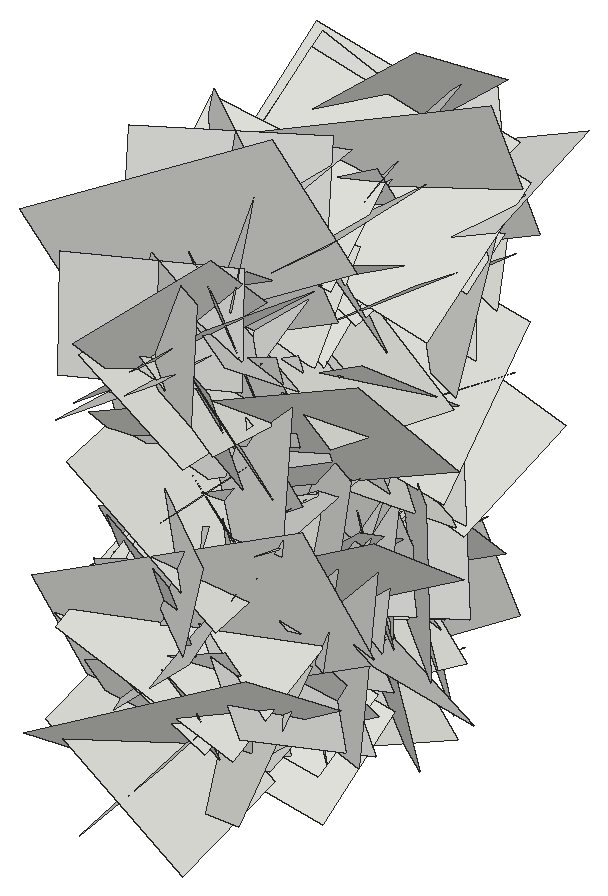
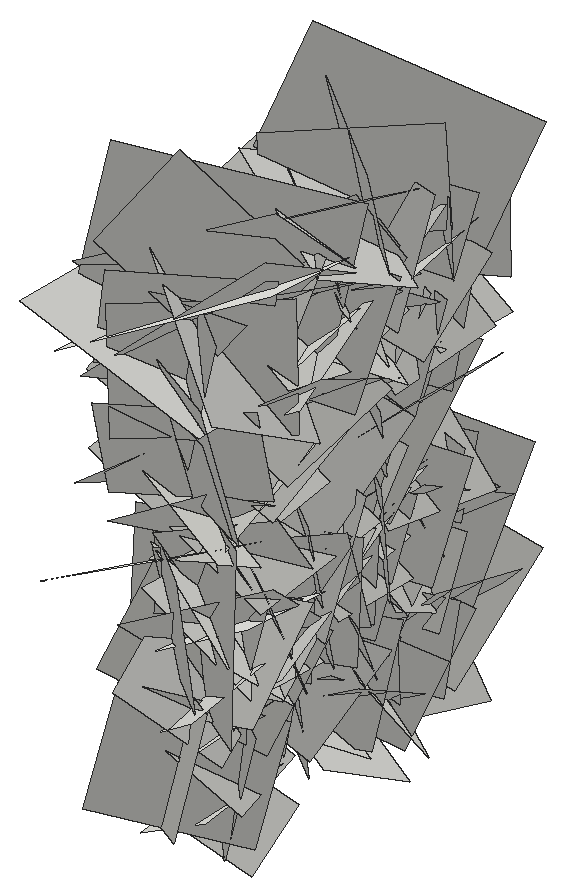
# SketchUp Ruby script. Lengths in inches.
U = 1.inch
M = Sketchup.active_model
def pt(a) = Geom::Point3d.new(a.map { |v| v * U })
def face(e, loops, mat)
  f = e.add_face(loops[0].map { |a| pt(a) })
  loops[1..].each { |l| e.add_face(l.map { |a| pt(a) }).erase! }
  f.material = f.back_material = mat if mat
  f
end
# faces: each face lists its corners as indices into pts; further lists are holes
def faces(e, pts, list, mat = nil) = list.each { |f| face(e, (f[0].is_a?(Array) ? f : [f]).map { |l| l.map { |i| pts[i] } }, mat) }
# xy, xz, yz: faces in a plane at the given z, y or x. An outline is a flat list of corners, or four numbers for a rectangle; further outlines are holes
def ring(l) = l.size == 4 ? [[l[0], l[1]], [l[2], l[1]], [l[2], l[3]], [l[0], l[3]]] : l.each_slice(2).to_a
def flat(e, list, mat, &to3) = list.each { |f| face(e, (f[0].is_a?(Array) ? f : [f]).map { |l| ring(l).map { |u, v| to3.(u, v) } }, mat) }
def xy(e, z, list, mat = nil) = flat(e, list, mat) { |x, y| [x, y, z] }
def xz(e, y, list, mat = nil) = flat(e, list, mat) { |x, z| [x, y, z] }
def yz(e, x, list, mat = nil) = flat(e, list, mat) { |y, z| [x, y, z] }
def lines(e, pts, list) = list.each { |a, b| e.add_line(pt(pts[a]), pt(pts[b])) }
# prism: a flat outline (further loops are holes) pulled along v
def prism(e, loops, v, mat = nil)
  f = face(e, loops, mat); d = Geom::Vector3d.new(v.map { |x| x * U })
  f.pushpull(f.normal.samedirection?(d) ? d.length : -d.length)
end
def box(e, o, s, mat = nil) = prism(e, [[o, [o[0] + s[0], o[1], o[2]], [o[0] + s[0], o[1] + s[1], o[2]], [o[0], o[1] + s[1], o[2]]]], [0, 0, s[2]], mat)
def at(x, y, z, deg = 0) = Geom::Transformation.translation(pt([x, y, z])) * Geom::Transformation.rotation(ORIGIN, Z_AXIS, deg.degrees)
def axes(o, x, y, z) = Geom::Transformation.new([*x, 0, *y, 0, *z, 0, *pt(o).to_a, 1])
def part(name) = M.definitions.add(name)
# library, detail: a bought-in or finely detailed component or shape, given as its bounding box
def library(name, o, s) = part(name).tap { |d| box(d.entities, o, s) }
def detail(e, o, s) = box(e.add_group.entities, o, s)
def put(e, d, t, mat = nil) = e.add_instance(d, t).tap { |i| i.material = mat if mat }
def group(e, t, mat = nil) = e.add_group.tap { |g| g.transformation = t; g.material = mat if mat }.entities
root = M.entities
c1 = part("Component\#6")
p = [[0.01,0,0],[0,3.24,4.54],[4.32,3.24,4.54],[4.33,0,0]]
faces(c1.entities,p,[[0,1,2,3]])
put(root,c1,axes([420.52,153.52,29.46],[-0.08102,0.00764,-0.81457],[-0.10707,-0.81193,0.00187],[0.85682,-0.10074,-0.07679]))
put(root,c1,axes([420.52,158.01,30.39],[0.08038,-0.60995,0.00551],[-0.02253,0.00291,0.6143],[0.64618,0.07598,0.02073]))
put(root,c1,axes([420.52,151.89,27.92],[0.07457,-0.37507,-0.49968],[-0.035,-0.50437,0.37394],[0.66135,0.0156,0.07613]))
put(root,c1,axes([424.49,158.65,23.12],[0.03,-0.65446,0.65644],[-0.11713,0.64968,0.65248],[-0.97555,-0.09812,-0.05816]))
put(root,c1,axes([420.52,150.81,32.67],[-0.03105,-0.70657,0.01303],[0.00041,0.01303,0.70717],[0.74909,-0.02929,0.00015]))
put(root,c1,axes([424.49,155.99,38.05],[-0.0315,0.52335,-0.79271],[0.01447,-0.79278,-0.52391],[-1.00678,-0.02777,0.01727]))
put(root,c1,axes([420.52,155.3,36.05],[-0.02231,-0.46484,-0.62566],[-0.10069,-0.6197,0.4636],[0.82005,-0.08874,0.0399]))
put(root,c1,axes([424.49,160.9375,37.33],[-0.13153,0.12633,-0.90974],[0.10231,-0.91113,-0.13969],[-0.96819,-0.11344,0.10882]))
put(root,c1,axes([424.49,153.79,24.7],[0.00565,-0.43188,0.90191],[0.04751,0.90112,0.43124],[-1.05892,0.03812,0.02416]))
put(root,c1,axes([424.49,152.27,30.34],[-0.04267,0.47891,-0.74389],[-0.05776,-0.74459,-0.47642],[-0.93603,0.02411,0.06331]))
put(root,c1,axes([424.49,150.92,33.45],[0.01124,-0.40239,0.85237],[-0.02564,0.85203,0.40253],[-0.99881,-0.0264,-0.00074]))
put(root,c1,axes([420.52,153.82,25.23],[0.04726,-0.11023,0.59197],[0.093,0.58845,0.10297],[0.63147,-0.07841,-0.05947]))
put(root,c1,axes([420.52,149.71,29.1],[0.04042,0.22115,-0.567],[0.10046,-0.56334,-0.21335],[0.63725,0.07479,0.0696]))
put(root,c1,axes([424.49,154.45,36.57],[-0.07713,0.81709,0.22722],[-0.03645,0.22503,-0.82021],[-0.89825,-0.07929,0.01378]))
put(root,c1,axes([420.52,158.75,26.14],[0.12859,0.59437,-0.23179],[-0.06253,-0.22448,-0.60651],[0.67335,-0.13435,-0.01206]))
put(root,c1,axes([424.49,156.72,22.08],[0.00521,-0.94479,0.50901],[0.17637,0.50353,0.93301],[-1.12382,0.07464,0.14878]))
put(root,c1,axes([420.52,156.34,37.48],[-0.20366,-0.78098,-0.33642],[0.07649,-0.35863,0.79133],[0.89812,-0.14656,-0.14368]))
put(root,c1,axes([424.49,150.56,37.37],[-0.01495,0.72639,-0.4873],[-0.06872,-0.48689,-0.7239],[-0.92463,0.02444,0.06168]))
put(root,c1,axes([420.52,156.49,28.09],[0.01227,0.36562,0.53928],[0.0952,0.53332,-0.36351],[0.68404,-0.08079,0.04092]))
put(root,c1,axes([424.49,150.4,30.92],[-0.04252,-0.27759,0.76161],[-0.13298,0.75548,0.26875],[-0.84891,-0.10444,-0.08025]))
put(root,c1,axes([424.49,152.31,24.83],[-0.14132,0.38772,0.61473],[-0.11706,0.60692,-0.40674],[-0.76145,-0.16526,-0.05156]))
put(root,c1,axes([420.52,150.69,21.46],[-0.08617,-0.06424,0.73191],[0.1147,0.7273,0.07585],[0.77031,-0.11548,0.07058]))
put(root,c1,axes([420.52,149.63,26.39],[-0.05575,0.3601,-0.58557],[0.15834,-0.56726,-0.36226],[0.71127,0.15451,0.03475]))
put(root,c1,axes([420.52,153.92,21.15],[-0.0271,-0.2919,0.8704],[-0.20523,0.85287,0.28034],[0.95124,0.17569,0.08528]))
put(root,c1,axes([420.52,159.1875,20.3125],[-0.01409,-0.35632,0.80543],[-0.16766,0.79339,0.34838],[0.91839,0.13938,0.07596]))
put(root,c1,axes([424.49,157.73,31.39],[0.13129,-0.92283,0.37392],[-0.04334,0.37177,0.93107],[-1.05456,-0.13017,0.00829]))
put(root,c1,axes([420.52,147.16,24.1],[-0.03025,0.92414,0.23442],[-0.23339,0.2218,-0.90118],[0.98329,0.08108,-0.20669]))
put(root,c1,axes([420.52,159.76,21.63],[0.09665,-0.666,0.12875],[-0.03078,0.12595,0.67212],[0.71837,0.095,0.01147]))
put(root,c1,axes([424.49,154.61,36.92],[0.07328,1.03426,0.55463],[0.26621,0.52968,-1.01904],[-1.21518,0.17841,-0.1898]))
put(root,c1,axes([420.52,160.84,30.26],[0.09118,-0.56201,-0.30691],[0.0596,-0.30185,0.56849],[0.67615,0.1024,-0.00872]))
put(root,c1,axes([420.52,156.05,22.34],[0.04217,-0.56806,-0.37659],[0.07293,-0.37196,0.56834],[0.71876,0.07107,-0.03557]))
put(root,c1,axes([424.49,158.82,28.52],[0.0834,-0.34729,-0.88838],[-0.00654,-0.89156,0.34799],[-1.01106,-0.02288,-0.07553]))
put(root,c1,axes([424.49,151.53,22],[0.08087,0.78957,0.40941],[-0.10212,0.41583,-0.78401],[-0.93722,0.02282,0.12075]))
put(root,c1,axes([424.49,152.86,25.21],[-0.07237,-0.84668,-0.40971],[0.16913,-0.41526,0.83156],[-0.98259,-0.00911,0.17331]))
put(root,c1,axes([424.49,150.44,37.52],[0.01758,-0.03984,-0.83316],[-0.08726,-0.82933,0.03802],[-0.87984,0.08145,-0.02042]))
put(root,c1,axes([424.49,161.57,34.4],[0.05292,-0.24359,-0.78611],[-0.1523,-0.77804,0.23197],[-0.85897,0.12294,-0.08956]))
put(root,c1,axes([420.52,154.14,39.875],[-0.07687,-0.17009,-0.90128],[-0.07958,-0.89996,0.17589],[0.96896,-0.0874,-0.05706]))
put(root,c1,axes([420.52,159.35,19.53],[0.12506,-0.65018,0.20227],[-0.00025,0.20525,0.65988],[0.72178,0.11273,-0.03482]))
put(root,c1,axes([424.49,155.63,34.51],[0.04715,-0.7148,-0.47013],[-0.06325,-0.47221,0.71232],[-0.90467,-0.00424,-0.0743]))
put(root,c1,axes([424.49,151.43,29.49],[0.01376,0.93036,0.01045],[0.09599,0.00914,-0.92605],[-0.98156,0.01394,-0.09041]))
put(root,c1,axes([424.49,156.02,27.27],[-0.01737,0.78195,0.05447],[-0.0729,0.05284,-0.77921],[-0.82768,-0.02106,0.06749]))
put(root,c1,axes([420.52,152.23,36.27],[0.17612,0.33723,0.58016],[-0.03508,0.60107,-0.33991],[0.71045,-0.05392,-0.16061]))
put(root,c1,axes([420.52,152.86,32.22],[-0.07765,-0.95123,0.12327],[-0.10469,0.13045,0.94796],[1.01133,-0.05954,0.1076]))
put(root,c1,axes([424.49,160.42,26.72],[0.04031,-0.6417,-0.5437],[-0.04231,-0.54502,0.64047],[-0.89052,-0.00315,-0.05504]))
put(root,c1,axes([420.52,153.18,27.99],[-0.08911,-1.01671,-0.11332],[-0.1646,-0.0997,1.00972],[1.07181,-0.09984,0.14565]))
put(root,c1,axes([424.49,153.18,27.99],[0.08911,-1.01671,-0.11332],[0.1646,-0.0997,1.00972],[-1.07181,-0.09984,0.14565]))
put(root,c1,axes([420.52,160.42,26.72],[-0.04031,-0.6417,-0.5437],[0.04231,-0.54502,0.64047],[0.89052,-0.00315,-0.05504]))
put(root,c1,axes([424.49,152.86,32.22],[0.07765,-0.95123,0.12327],[0.10469,0.13045,0.94796],[-1.01133,-0.05954,0.1076]))
put(root,c1,axes([424.49,152.23,36.27],[-0.17612,0.33723,0.58016],[0.03508,0.60107,-0.33991],[-0.71045,-0.05392,-0.16061]))
put(root,c1,axes([420.52,156.02,27.27],[0.01737,0.78195,0.05447],[0.0729,0.05284,-0.77921],[0.82768,-0.02106,0.06749]))
put(root,c1,axes([420.52,151.43,29.49],[-0.01376,0.93036,0.01045],[-0.09599,0.00914,-0.92605],[0.98156,0.01394,-0.09041]))
put(root,c1,axes([420.52,155.63,34.51],[-0.04715,-0.7148,-0.47013],[0.06325,-0.47221,0.71232],[0.90467,-0.00424,-0.0743]))
put(root,c1,axes([424.49,159.35,19.53],[-0.12506,-0.65018,0.20227],[0.00025,0.20525,0.65988],[-0.72178,0.11273,-0.03482]))
put(root,c1,axes([424.49,154.14,39.875],[0.07687,-0.17009,-0.90128],[0.07958,-0.89996,0.17589],[-0.96896,-0.0874,-0.05706]))
put(root,c1,axes([420.52,161.57,34.4],[-0.05292,-0.24359,-0.78611],[0.1523,-0.77804,0.23197],[0.85897,0.12294,-0.08956]))
put(root,c1,axes([420.52,150.44,37.52],[-0.01758,-0.03984,-0.83316],[0.08726,-0.82933,0.03802],[0.87984,0.08145,-0.02042]))
put(root,c1,axes([420.52,152.86,25.21],[0.07237,-0.84668,-0.40971],[-0.16913,-0.41526,0.83156],[0.98259,-0.00911,0.17331]))
put(root,c1,axes([420.52,151.53,22],[-0.08087,0.78957,0.40941],[0.10212,0.41583,-0.78401],[0.93722,0.02282,0.12075]))
put(root,c1,axes([420.52,158.82,28.52],[-0.0834,-0.34729,-0.88838],[0.00654,-0.89156,0.34799],[1.01106,-0.02288,-0.07553]))
put(root,c1,axes([424.49,156.05,22.34],[-0.04217,-0.56806,-0.37659],[-0.07293,-0.37196,0.56834],[-0.71876,0.07107,-0.03557]))
put(root,c1,axes([424.49,160.84,30.26],[-0.09118,-0.56201,-0.30691],[-0.0596,-0.30185,0.56849],[-0.67615,0.1024,-0.00872]))
put(root,c1,axes([420.52,154.61,36.92],[-0.07328,1.03426,0.55463],[-0.26621,0.52968,-1.01904],[1.21518,0.17841,-0.1898]))
put(root,c1,axes([424.49,159.76,21.63],[-0.09665,-0.666,0.12875],[0.03078,0.12595,0.67212],[-0.71837,0.095,0.01147]))
put(root,c1,axes([424.49,147.16,24.1],[0.03025,0.92414,0.23442],[0.23339,0.2218,-0.90118],[-0.98329,0.08108,-0.20669]))
put(root,c1,axes([420.52,157.73,31.39],[-0.13129,-0.92283,0.37392],[0.04334,0.37177,0.93107],[1.05456,-0.13017,0.00829]))
put(root,c1,axes([424.49,159.1875,20.3125],[0.01409,-0.35632,0.80543],[0.16766,0.79339,0.34838],[-0.91839,0.13938,0.07596]))
put(root,c1,axes([424.49,153.92,21.15],[0.0271,-0.2919,0.8704],[0.20523,0.85287,0.28034],[-0.95124,0.17569,0.08528]))
put(root,c1,axes([424.49,149.63,26.39],[0.05575,0.3601,-0.58557],[-0.15834,-0.56726,-0.36226],[-0.71127,0.15451,0.03475]))
put(root,c1,axes([424.49,150.69,21.46],[0.08617,-0.06424,0.73191],[-0.1147,0.7273,0.07585],[-0.77031,-0.11548,0.07058]))
put(root,c1,axes([420.52,152.31,24.83],[0.14132,0.38772,0.61473],[0.11706,0.60692,-0.40674],[0.76145,-0.16526,-0.05156]))
put(root,c1,axes([420.52,150.4,30.92],[0.04252,-0.27759,0.76161],[0.13298,0.75548,0.26875],[0.84891,-0.10444,-0.08025]))
put(root,c1,axes([424.49,156.49,28.09],[-0.01227,0.36562,0.53928],[-0.0952,0.53332,-0.36351],[-0.68404,-0.08079,0.04092]))
put(root,c1,axes([420.52,150.56,37.37],[0.01495,0.72639,-0.4873],[0.06872,-0.48689,-0.7239],[0.92463,0.02444,0.06168]))
put(root,c1,axes([424.49,156.34,37.48],[0.20366,-0.78098,-0.33642],[-0.07649,-0.35863,0.79133],[-0.89812,-0.14656,-0.14368]))
put(root,c1,axes([420.52,156.72,22.08],[-0.00521,-0.94479,0.50901],[-0.17637,0.50353,0.93301],[1.12382,0.07464,0.14878]))
put(root,c1,axes([424.49,158.75,26.14],[-0.12859,0.59437,-0.23179],[0.06253,-0.22448,-0.60651],[-0.67335,-0.13435,-0.01206]))
put(root,c1,axes([420.52,154.45,36.57],[0.07713,0.81709,0.22722],[0.03645,0.22503,-0.82021],[0.89825,-0.07929,0.01378]))
put(root,c1,axes([424.49,149.71,29.1],[-0.04042,0.22115,-0.567],[-0.10046,-0.56334,-0.21335],[-0.63725,0.07479,0.0696]))
put(root,c1,axes([424.49,153.82,25.23],[-0.04726,-0.11023,0.59197],[-0.093,0.58845,0.10297],[-0.63147,-0.07841,-0.05947]))
put(root,c1,axes([420.52,150.92,33.45],[-0.01124,-0.40239,0.85237],[0.02564,0.85203,0.40253],[0.99881,-0.0264,-0.00074]))
put(root,c1,axes([420.52,152.27,30.34],[0.04267,0.47891,-0.74389],[0.05776,-0.74459,-0.47642],[0.93603,0.02411,0.06331]))
put(root,c1,axes([420.52,153.79,24.7],[-0.00565,-0.43188,0.90191],[-0.04751,0.90112,0.43124],[1.05892,0.03812,0.02416]))
put(root,c1,axes([420.52,160.9375,37.33],[0.13153,0.12633,-0.90974],[-0.10231,-0.91113,-0.13969],[0.96819,-0.11344,0.10882]))
put(root,c1,axes([424.49,155.3,36.05],[0.02231,-0.46484,-0.62566],[0.10069,-0.6197,0.4636],[-0.82005,-0.08874,0.0399]))
put(root,c1,axes([420.52,155.99,38.05],[0.0315,0.52335,-0.79271],[-0.01447,-0.79278,-0.52391],[1.00678,-0.02777,0.01727]))
put(root,c1,axes([424.49,150.81,32.67],[0.03105,-0.70657,0.01303],[-0.00041,0.01303,0.70717],[-0.74909,-0.02929,0.00015]))
put(root,c1,axes([420.52,158.65,23.12],[-0.03,-0.65446,0.65644],[0.11713,0.64968,0.65248],[0.97555,-0.09812,-0.05816]))
put(root,c1,axes([424.49,151.89,27.92],[-0.07457,-0.37507,-0.49968],[0.035,-0.50437,0.37394],[-0.66135,0.0156,0.07613]))
put(root,c1,axes([424.49,158.01,30.39],[-0.08038,-0.60995,0.00551],[0.02253,0.00291,0.6143],[-0.64618,0.07598,0.02073]))
put(root,c1,axes([424.49,153.52,29.46],[0.08102,0.00764,-0.81457],[0.10707,-0.81193,0.00187],[-0.85682,-0.10074,-0.07679]))
put(root,c1,axes([420.52,152.65,32.7],[-0.31384,1.21799,0.62272],[-0.13011,0.61092,-1.25326],[1.44417,0.31973,0.02242]))
put(root,c1,axes([420.52,149.65,34.23],[-0.2234,-0.54463,1.08834],[-0.02633,1.10624,0.54877],[1.28976,-0.07175,0.19972]))
put(root,c1,axes([424.49,152.7,33.94],[0.15183,0.13661,-0.74127],[-0.04087,-0.75222,-0.14607],[-0.79793,0.06452,-0.13357]))
put(root,c1,axes([424.49,158.73,27.09],[0.13155,-0.14233,-0.74779],[0.00006,-0.75766,0.14422],[-0.80689,-0.02326,-0.12191]))
put(root,c1,axes([420.52,158.66,27.8],[0.19419,0.10037,-0.91545],[-0.10975,-0.92523,-0.12216],[0.97001,-0.12478,0.16945]))
put(root,c1,axes([424.49,156.65,23.33],[-0.01341,0.01203,0.69899],[0.10657,0.69187,-0.01009],[-0.73333,0.10033,-0.01425]))
put(root,c1,axes([420.52,154.96,37.56],[-0.27688,1.1515,0.31839],[0.11464,0.34737,-1.16756],[1.26119,0.22122,0.17603]))
put(root,c1,axes([420.52,152.42,20.54],[-0.05004,-0.6691,0.77955],[0.05919,0.77755,0.67076],[1.08735,-0.07312,-0.00064]))
put(root,c1,axes([424.49,161,38.46],[0.19651,-0.13504,-0.81499],[0.03185,-0.8336,0.14496],[-0.87508,-0.06067,-0.17773]))
put(root,c1,axes([420.52,159.15,23.91],[0.14407,0.13595,-0.90237],[-0.02833,-0.91134,-0.14133],[0.9669,-0.04696,0.13032]))
put(root,c1,axes([420.52,151.25,34.8],[0.16779,0.3958,-0.75565],[0.05631,-0.77163,-0.39305],[0.90246,-0.02545,0.16502]))
put(root,c1,axes([424.49,158.03,24.73],[0.19324,-0.05037,0.89121],[0.15909,0.89838,0.02008],[-0.93272,0.1428,0.18806]))
put(root,c1,axes([420.52,154.4,23.625],[-0.0407,-0.65785,-0.83395],[0.03781,-0.83482,0.65689],[1.12528,0.00426,-0.05223]))
put(root,c1,axes([424.49,157.59,40.82],[0.16311,0.68993,-0.43022],[0.09586,-0.44966,-0.68876],[-0.85651,0.08106,-0.15901]))
put(root,c1,axes([420.52,154.59,24.16],[-0.1724,0.15274,1.09758],[0.17194,1.10067,-0.12914],[1.16199,-0.14021,0.18195]))
put(root,c1,axes([420.52,152.14,28.92],[0.00837,0.82237,-0.50147],[0.16225,-0.49618,-0.8113],[1.00803,0.07304,0.13474]))
put(root,c1,axes([424.49,149.08,38.35],[-0.0057,0.54335,-0.52891],[0.23788,-0.50408,-0.52014],[-0.76776,-0.16022,-0.15723]))
put(root,c1,axes([424.49,157.4,31.875],[0.05779,-0.51798,-0.36432],[0.0587,-0.36037,0.52065],[-0.6687,-0.0764,0.01422]))
put(root,c1,axes([420.52,156.45,32.24],[0.14884,0.843,-0.57449],[-0.06248,-0.57223,-0.85409],[1.07954,-0.14935,0.02978]))
put(root,c1,axes([424.49,160.09,33.87],[0.13785,-0.16653,-0.67513],[0.04892,-0.68326,0.17743],[-0.73546,-0.07666,-0.11474]))
put(root,c1,axes([420.52,156.02,28.65],[-0.0619,-0.85924,0.62732],[0.17366,0.61351,0.85557],[1.11425,-0.14335,-0.09849]))
put(root,c1,axes([424.49,147.9,27.03],[0.12769,0.03013,0.63893],[0.01482,0.64988,-0.03329],[-0.67785,0.01989,0.11963]))
put(root,c1,axes([420.52,156.69,29.48],[-0.02364,1.01192,0.31394],[0.16386,0.31376,-1.00035],[1.11105,-0.02474,0.15421]))
put(root,c1,axes([420.52,161.68,35.57],[-0.09547,-0.29138,-1.10436],[0.14499,-1.10257,0.27976],[1.20197,0.10985,-0.12146]))
put(root,c1,axes([420.52,147.58,26.68],[0.22766,0.71104,0.67114],[-0.02672,0.69094,-0.72395],[1.03608,-0.13842,-0.16614]))
put(root,c1,axes([420.52,153.43,27.14],[0.15407,-0.97446,-0.01303],[0.08051,-0.00181,0.98239],[1.02988,0.14592,-0.07485]))
put(root,c1,axes([420.52,158.93,27.77],[-0.0679,-1.16178,0.21088],[0.08573,0.20637,1.16154],[1.24867,-0.07734,-0.06828]))
put(root,c1,axes([420.52,160.05,30.35],[-0.12426,0.20575,-1.35522],[-0.11745,-1.35714,-0.19646],[1.44825,-0.0924,-0.13221]))
put(root,c1,axes([420.52,157.84,26.69],[0.16666,-0.37984,-0.88441],[0.10341,-0.88523,0.39754],[1.01503,0.15255,0.10471]))
put(root,c1,axes([420.52,153.58,31.99],[0.17505,-0.32324,-0.90395],[0.10086,-0.9072,0.34179],[1.0126,0.14624,0.12223]))
put(root,c1,axes([420.52,151.45,29.33],[0.11063,1.17252,-0.59491],[-0.28501,-0.56514,-1.16101],[1.36425,-0.21315,-0.19431]))
put(root,c1,axes([420.52,155.57,33.875],[0.13701,-1.11756,0.11199],[-0.07264,0.10468,1.12363],[1.18833,0.13525,0.05577]))
put(root,c1,axes([420.52,156.79,29.67],[0.01777,-0.29003,-1.18393],[-0.05362,-1.18318,0.28913],[1.29096,-0.04516,0.0283]))
put(root,c1,axes([420.52,158.37,30.5],[0.12568,-1.12455,0.31778],[-0.06348,0.31314,1.13049],[1.23707,0.13032,0.02572]))
put(root,c1,axes([420.52,152.25,36.24],[-0.0137,1.21221,-0.26433],[0.01965,-0.26413,-1.21218],[1.31499,0.01657,0.01536]))
put(root,c1,axes([420.52,150.2,21.48],[0.03659,-0.96074,0.6365],[0.08804,0.6372,0.9573],[1.21843,-0.01719,-0.08829]))
put(root,c1,axes([420.52,149.67,23.37],[-0.09539,-0.59855,1.14231],[0.08783,1.14003,0.60389],[1.36418,-0.11525,0.041]))
put(root,c1,axes([420.52,153.92,36.42],[0.14295,0.82362,0.79821],[0.11339,0.79118,-0.83443],[1.21047,-0.17138,-0.0161]))
put(root,c1,axes([420.52,156.14,33.68],[0.06217,-0.55405,1.15944],[0.03014,1.16092,0.55332],[1.36179,-0.0004,-0.06518]))
put(root,c1,axes([420.52,157.5625,26.25],[0.15158,-0.38022,-1.22414],[-0.0526,-1.23246,0.37701],[1.35773,-0.0053,0.15127]))
put(root,c1,axes([420.52,161.74,34.71],[0.1652,-1.10091,-0.16395],[0.26327,-0.12698,1.08875],[1.15009,0.1872,-0.22568]))
put(root,c1,axes([420.52,153.73,28.3],[-0.01858,0.99462,-0.84655],[0.29457,-0.8244,-0.97435],[1.35277,0.19318,0.20054]))
put(root,c1,axes([420.52,153.125,28.17],[-0.03085,-0.9293,0.97672],[0.26234,0.95667,0.91759],[1.40479,-0.19906,-0.14991]))
put(root,c1,axes([420.52,153.14,23.91],[0.18,-1.08552,0.79109],[0.08355,0.80406,1.08641],[1.42134,0.0902,-0.16405]))
